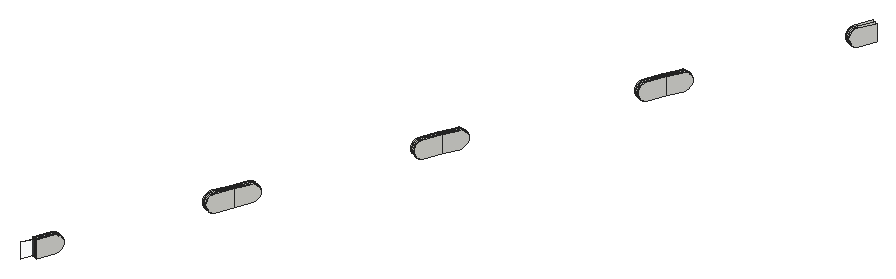
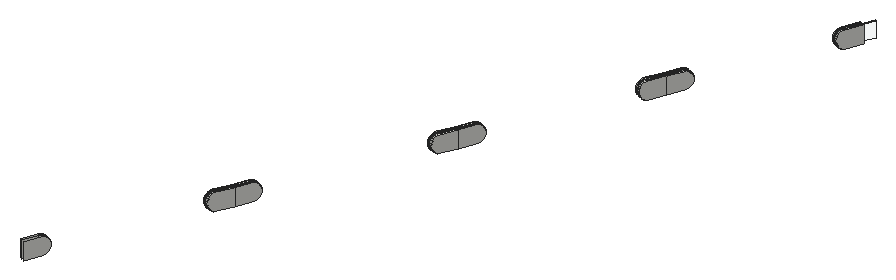
# SketchUp Ruby script. Lengths in inches.
U = 1.inch
M = Sketchup.active_model
def pt(a) = Geom::Point3d.new(a.map { |v| v * U })
def face(e, loops, mat)
  f = e.add_face(loops[0].map { |a| pt(a) })
  loops[1..].each { |l| e.add_face(l.map { |a| pt(a) }).erase! }
  f.material = f.back_material = mat if mat
  f
end
# faces: each face lists its corners as indices into pts; further lists are holes
def faces(e, pts, list, mat = nil) = list.each { |f| face(e, (f[0].is_a?(Array) ? f : [f]).map { |l| l.map { |i| pts[i] } }, mat) }
# xy, xz, yz: faces in a plane at the given z, y or x. An outline is a flat list of corners, or four numbers for a rectangle; further outlines are holes
def ring(l) = l.size == 4 ? [[l[0], l[1]], [l[2], l[1]], [l[2], l[3]], [l[0], l[3]]] : l.each_slice(2).to_a
def flat(e, list, mat, &to3) = list.each { |f| face(e, (f[0].is_a?(Array) ? f : [f]).map { |l| ring(l).map { |u, v| to3.(u, v) } }, mat) }
def xy(e, z, list, mat = nil) = flat(e, list, mat) { |x, y| [x, y, z] }
def xz(e, y, list, mat = nil) = flat(e, list, mat) { |x, z| [x, y, z] }
def yz(e, x, list, mat = nil) = flat(e, list, mat) { |y, z| [x, y, z] }
def lines(e, pts, list) = list.each { |a, b| e.add_line(pt(pts[a]), pt(pts[b])) }
# prism: a flat outline (further loops are holes) pulled along v
def prism(e, loops, v, mat = nil)
  f = face(e, loops, mat); d = Geom::Vector3d.new(v.map { |x| x * U })
  f.pushpull(f.normal.samedirection?(d) ? d.length : -d.length)
end
def box(e, o, s, mat = nil) = prism(e, [[o, [o[0] + s[0], o[1], o[2]], [o[0] + s[0], o[1] + s[1], o[2]], [o[0], o[1] + s[1], o[2]]]], [0, 0, s[2]], mat)
def at(x, y, z, deg = 0) = Geom::Transformation.translation(pt([x, y, z])) * Geom::Transformation.rotation(ORIGIN, Z_AXIS, deg.degrees)
def axes(o, x, y, z) = Geom::Transformation.new([*x, 0, *y, 0, *z, 0, *pt(o).to_a, 1])
def part(name) = M.definitions.add(name)
# library, detail: a bought-in or finely detailed component or shape, given as its bounding box
def library(name, o, s) = part(name).tap { |d| box(d.entities, o, s) }
def detail(e, o, s) = box(e.add_group.entities, o, s)
def put(e, d, t, mat = nil) = e.add_instance(d, t).tap { |i| i.material = mat if mat }
def group(e, t, mat = nil) = e.add_group.tap { |g| g.transformation = t; g.material = mat if mat }.entities
root = M.entities
M.materials.add("Glass_Safety_01").color = [204, 235, 244]
M.materials["Glass_Safety_01"].alpha = 0.1
xy(root,333,[[908.41,684.63,908.15,684.74,908.9375,686.55,909.19,686.4375],[907.97,684.82,907.72,684.93,908.51,686.74,908.76,686.625],[916.34,702.85,916.09,702.96,916.16,703.12,916.87,704.76,917.125,704.65],[915.91,703.04,915.65,703.15,916.4375,704.95,916.69,704.84,915.98,703.2],[917.125,704.65,916.87,704.76,917.66,706.57,917.91,706.46],
  [916.69,704.84,916.4375,704.95,917.23,706.76,917.48,706.65],[925.57,724.04,925.32,724.15,925.38,724.31,926.1,725.96,926.36,725.85],[925.14,724.23,924.88,724.34,925.67,726.15,925.92,726.04,925.2,724.39],[926.36,725.85,926.1,725.96,926.89,727.76,927.14,727.65],[925.92,726.04,925.67,726.15,926.46,727.95,926.71,727.84],
  [935.5,746.83,935.24,746.94,935.3,747.08,936.03,748.75,936.28,748.64],[935.0625,747.02,934.81,747.13,935.6,748.94,935.85,748.83,935.125,747.16],[936.28,748.64,936.03,748.75,936.82,750.55,937.07,750.4375],[935.85,748.83,935.6,748.94,936.39,750.74,936.64,750.63]])
xy(root,333.08,[[908.15,684.74,907.97,684.82,908.6,686.26,908.78,686.1875],[916.24,703.32,916.0625,703.4,916.69,704.84,916.87,704.76],[916.87,704.76,916.69,704.84,917.32,706.28,917.5,706.21],[925.47,724.51,925.29,724.59,925.92,726.04,926.1,725.96],[926.1,725.96,925.92,726.04,926.55,727.48,926.73,727.4],
  [935.4,747.3,935.22,747.38,935.85,748.83,935.9375,748.79,936.03,748.75],[936.03,748.75,935.9375,748.79,935.85,748.83,936.48,750.27,936.66,750.1875]],"Glass_Safety_01")
xy(root,335.05,[[907.52,683.3,908.15,684.74,907.97,684.82,907.34,683.375],[908.15,684.74,908.78,686.1875,908.6,686.26,907.97,684.82],[916.24,703.32,916.87,704.76,916.69,704.84,916.0625,703.4],[916.87,704.76,917.5,706.21,917.32,706.28,916.69,704.84],[925.47,724.51,926.1,725.96,925.92,726.04,925.29,724.59],
  [926.1,725.96,926.73,727.4,926.55,727.48,925.92,726.04],[935.4,747.3,936.03,748.75,935.9375,748.79,935.85,748.83,935.22,747.38],[936.03,748.75,936.66,750.1875,936.48,750.27,935.85,748.83,935.9375,748.79]],"Glass_Safety_01")
xy(root,335.125,[[908.41,684.63,909.19,686.4375,908.9375,686.55,908.15,684.74],[907.97,684.82,908.76,686.625,908.51,686.74,907.72,684.93],[916.34,702.85,917.125,704.65,916.87,704.76,916.16,703.12,916.09,702.96],[915.91,703.04,915.98,703.2,916.69,704.84,916.4375,704.95,915.65,703.15],[917.125,704.65,917.91,706.46,917.66,706.57,916.87,704.76],
  [916.69,704.84,917.48,706.65,917.23,706.76,916.4375,704.95],[925.57,724.04,926.36,725.85,926.1,725.96,925.38,724.31,925.32,724.15],[925.14,724.23,925.2,724.39,925.92,726.04,925.67,726.15,924.88,724.34],[926.36,725.85,927.14,727.65,926.89,727.76,926.1,725.96],[925.92,726.04,926.71,727.84,926.46,727.95,925.67,726.15],
  [935.5,746.83,936.28,748.64,936.03,748.75,935.3,747.08,935.24,746.94],[935.0625,747.02,935.125,747.16,935.85,748.83,935.6,748.94,934.81,747.13],[936.28,748.64,937.07,750.4375,936.82,750.55,936.03,748.75],[935.85,748.83,936.64,750.63,936.39,750.74,935.6,748.94]])
p = [[908.15,684.74,333],[908.15,684.74,333.08],[908.15,684.74,335.05],[908.15,684.74,335.125],[908.41,684.63,335.125],[908.41,684.63,333],
  [909.19,686.4375,335.125],[909.19,686.4375,333],[909.3,686.6875,333.04],[909.4,686.92,333.14],[909.49,687.125,333.3125],[909.56,687.28,333.53],
  [909.6,687.38,333.79],[909.62,687.41,334.0625],[909.6,687.38,334.34],[909.56,687.28,334.59],[909.49,687.125,334.8125],[909.4,686.92,334.98],
  [909.3,686.6875,335.09],[908.9375,686.55,335.125],[908.9375,686.55,333],[908.78,686.1875,333.08],[908.78,686.1875,335.05],[907.97,684.82,333.08],
  [907.97,684.82,333],[907.72,684.93,333],[907.72,684.93,335.125],[907.97,684.82,335.125],[907.97,684.82,335.05],[908.76,686.625,333],
  [908.76,686.625,335.125],[908.6,686.26,335.05],[908.6,686.26,333.08],[908.51,686.74,335.125],[908.62,686.99,335.09],[908.72,687.22,334.98],
  [908.81,687.42,334.8125],[908.875,687.58,334.59],[908.92,687.68,334.34],[908.93,687.71,334.0625],[908.92,687.68,333.79],[908.875,687.58,333.53],
  [908.81,687.42,333.3125],[908.72,687.22,333.14],[908.62,686.99,333.04],[908.51,686.74,333],[909.05,686.8,333.04],[909.15,687.03,333.14],
  [909.24,687.24,333.3125],[909.31,687.39,333.53],[909.35,687.49,333.79],[909.36,687.52,334.0625],[909.35,687.49,334.34],[909.31,687.39,334.59],
  [909.24,687.24,334.8125],[909.15,687.03,334.98],[909.05,686.8,335.09],[908.87,686.88,333.04],[908.87,686.88,335.09],[908.97,687.11,334.98],
  [909.06,687.3125,334.8125],[909.125,687.47,334.59],[909.17,687.57,334.34],[909.18,687.6,334.0625],[909.17,687.57,333.79],[909.125,687.47,333.53],
  [909.06,687.3125,333.3125],[908.97,687.11,333.14],[917.125,704.65,335.125],[916.34,702.85,335.125],[916.23,702.6,335.09],[916.125,702.36,334.98],
  [916.04,702.16,334.8125],[915.97,702,334.59],[915.93,701.91,334.34],[915.91,701.875,334.0625],[915.93,701.91,333.79],[915.97,702,333.53],
  [916.04,702.16,333.3125],[916.125,702.36,333.14],[916.23,702.6,333.04],[916.34,702.85,333],[917.125,704.65,333],[916.09,702.96,335.125],
  [916.16,703.12,335.125],[916.16,703.12,333],[916.09,702.96,333],[915.98,702.71,333.04],[915.875,702.47,333.14],[915.79,702.27,333.3125],
  [915.72,702.11,333.53],[915.68,702.02,333.79],[915.66,701.98,334.0625],[915.68,702.02,334.34],[915.72,702.11,334.59],[915.79,702.27,334.8125],
  [915.875,702.47,334.98],[915.98,702.71,335.09],[915.91,703.04,333],[915.98,703.2,333],[915.98,703.2,335.125],[915.91,703.04,335.125],
  [915.8,702.78,335.09],[915.69,702.55,334.98],[915.61,702.35,334.8125],[915.54,702.19,334.59],[915.5,702.1,334.34],[915.48,702.0625,334.0625],
  [915.5,702.1,333.79],[915.54,702.19,333.53],[915.61,702.35,333.3125],[915.69,702.55,333.14],[915.8,702.78,333.04],[915.65,703.15,335.125],
  [916.4375,704.95,335.125],[916.4375,704.95,333],[915.65,703.15,333],[915.54,702.89,333.04],[915.44,702.66,333.14],[915.35,702.46,333.3125],
  [915.29,702.3,333.53],[915.24,702.21,333.79],[915.23,702.17,334.0625],[915.24,702.21,334.34],[915.29,702.3,334.59],[915.35,702.46,334.8125],
  [915.44,702.66,334.98],[915.54,702.89,335.09],[916.87,704.76,333],[916.87,704.76,335.125],[916.87,704.76,335.05],[916.24,703.32,335.05],
  [916.24,703.32,333.08],[916.87,704.76,333.08],[916.69,704.84,335.125],[916.69,704.84,333],[916.69,704.84,333.08],[916.0625,703.4,333.08],
  [916.0625,703.4,335.05],[916.69,704.84,335.05],[917.91,706.46,335.125],[917.91,706.46,333],[918.02,706.71,333.04],[918.125,706.94,333.14],
  [918.21,707.15,333.3125],[918.28,707.3,333.53],[918.32,707.4,333.79],[918.34,707.43,334.0625],[918.32,707.4,334.34],[918.28,707.3,334.59],
  [918.21,707.15,334.8125],[918.125,706.94,334.98],[918.02,706.71,335.09],[917.48,706.65,333],[917.48,706.65,335.125],[917.32,706.28,335.05],
  [917.32,706.28,333.08],[917.66,706.57,335.125],[917.66,706.57,333],[917.5,706.21,333.08],[917.5,706.21,335.05],[917.23,706.76,335.125],
  [917.33,707.01,335.09],[917.4375,707.24,334.98],[917.53,707.45,334.8125],[917.59,707.6,334.59],[917.64,707.7,334.34],[917.65,707.73,334.0625],
  [917.64,707.7,333.79],[917.59,707.6,333.53],[917.53,707.45,333.3125],[917.4375,707.24,333.14],[917.33,707.01,333.04],[917.23,706.76,333],
  [917.77,706.82,333.04],[917.59,706.9,333.04],[917.59,706.9,335.09],[917.69,707.13,334.98],[917.78,707.34,334.8125],[917.85,707.49,334.59],
  [917.89,707.59,334.34],[917.9,707.62,334.0625],[917.89,707.59,333.79],[917.85,707.49,333.53],[917.78,707.34,333.3125],[917.69,707.13,333.14],
  [917.87,707.05,333.14],[917.96,707.26,333.3125],[918.03,707.41,333.53],[918.07,707.51,333.79],[918.08,707.54,334.0625],[918.07,707.51,334.34],
  [918.03,707.41,334.59],[917.96,707.26,334.8125],[917.87,707.05,334.98],[917.77,706.82,335.09],[926.36,725.85,335.125],[925.57,724.04,335.125],
  [925.46,723.79,335.09],[925.36,723.56,334.98],[925.27,723.35,334.8125],[925.2,723.2,334.59],[925.16,723.1,334.34],[925.15,723.07,334.0625],
  [925.16,723.1,333.79],[925.2,723.2,333.53],[925.27,723.35,333.3125],[925.36,723.56,333.14],[925.46,723.79,333.04],[925.57,724.04,333],
  [926.36,725.85,333],[925.32,724.15,335.125],[925.38,724.31,335.125],[925.38,724.31,333],[925.32,724.15,333],[925.21,723.9,333.04],
  [925.11,723.67,333.14],[925.02,723.46,333.3125],[924.95,723.31,333.53],[924.91,723.21,333.79],[924.89,723.18,334.0625],[924.91,723.21,334.34],
  [924.95,723.31,334.59],[925.02,723.46,334.8125],[925.11,723.67,334.98],[925.21,723.9,335.09],[925.14,724.23,333],[925.2,724.39,333],
  [925.2,724.39,335.125],[925.14,724.23,335.125],[925.03,723.98,335.09],[924.92,723.74,334.98],[924.84,723.54,334.8125],[924.77,723.39,334.59],
  [924.73,723.29,334.34],[924.71,723.26,334.0625],[924.73,723.29,333.79],[924.77,723.39,333.53],[924.84,723.54,333.3125],[924.92,723.74,333.14],
  [925.03,723.98,333.04],[924.88,724.34,335.125],[925.67,726.15,335.125],[925.67,726.15,333],[924.88,724.34,333],[924.77,724.09,333.04],
  [924.67,723.85,333.14],[924.58,723.65,333.3125],[924.52,723.5,333.53],[924.47,723.4,333.79],[924.46,723.37,334.0625],[924.47,723.4,334.34],
  [924.52,723.5,334.59],[924.58,723.65,334.8125],[924.67,723.85,334.98],[924.77,724.09,335.09],[926.1,725.96,333],[926.1,725.96,335.125],
  [926.1,725.96,335.05],[925.47,724.51,335.05],[925.47,724.51,333.08],[926.1,725.96,333.08],[925.92,726.04,335.125],[925.92,726.04,333],
  [925.92,726.04,333.08],[925.29,724.59,333.08],[925.29,724.59,335.05],[925.92,726.04,335.05],[927.14,727.65,335.125],[927.14,727.65,333],
  [927.25,727.91,333.04],[927.35,728.14,333.14],[927.44,728.34,333.3125],[927.51,728.5,333.53],[927.55,728.59,333.79],[927.57,728.63,334.0625],
  [927.55,728.59,334.34],[927.51,728.5,334.59],[927.44,728.34,334.8125],[927.35,728.14,334.98],[927.25,727.91,335.09],[926.71,727.84,333],
  [926.71,727.84,335.125],[926.55,727.48,335.05],[926.55,727.48,333.08],[926.89,727.76,335.125],[926.89,727.76,333],[926.73,727.4,333.08],
  [926.73,727.4,335.05],[926.46,727.95,335.125],[926.57,728.2,335.09],[926.67,728.4375,334.98],[926.76,728.64,334.8125],[926.82,728.8,334.59],
  [926.87,728.89,334.34],[926.88,728.93,334.0625],[926.87,728.89,333.79],[926.82,728.8,333.53],[926.76,728.64,333.3125],[926.67,728.4375,333.14],
  [926.57,728.2,333.04],[926.46,727.95,333],[927,728.02,333.04],[926.82,728.09,333.04],[926.82,728.09,335.09],[926.92,728.33,334.98],
  [927.01,728.53,334.8125],[927.08,728.6875,334.59],[927.12,728.78,334.34],[927.13,728.82,334.0625],[927.12,728.78,333.79],[927.08,728.6875,333.53],
  [927.01,728.53,333.3125],[926.92,728.33,333.14],[927.1,728.25,333.14],[927.19,728.45,333.3125],[927.26,728.61,333.53],[927.3,728.7,333.79],
  [927.3125,728.74,334.0625],[927.3,728.7,334.34],[927.26,728.61,334.59],[927.19,728.45,334.8125],[927.1,728.25,334.98],[927,728.02,335.09],
  [936.28,748.64,335.125],[935.5,746.83,335.125],[935.39,746.58,335.09],[935.28,746.34,334.98],[935.2,746.14,334.8125],[935.13,745.99,334.59],
  [935.09,745.89,334.34],[935.07,745.86,334.0625],[935.09,745.89,333.79],[935.13,745.99,333.53],[935.2,746.14,333.3125],[935.28,746.34,333.14],
  [935.39,746.58,333.04],[935.5,746.83,333],[936.28,748.64,333],[935.0625,747.02,333],[935.125,747.16,333],[935.125,747.16,335.125],
  [935.0625,747.02,335.125],[934.95,746.77,335.09],[934.85,746.53,334.98],[934.76,746.33,334.8125],[934.69,746.18,334.59],[934.65,746.08,334.34],
  [934.64,746.05,334.0625],[934.65,746.08,333.79],[934.69,746.18,333.53],[934.76,746.33,333.3125],[934.85,746.53,333.14],[934.95,746.77,333.04],
  [935.24,746.94,335.125],[935.3,747.08,335.125],[935.3,747.08,333],[935.24,746.94,333],[935.13,746.69,333.04],[935.03,746.45,333.14],
  [934.94,746.25,333.3125],[934.875,746.1,333.53],[934.83,746,333.79],[934.82,745.97,334.0625],[934.83,746,334.34],[934.875,746.1,334.59],
  [934.94,746.25,334.8125],[935.03,746.45,334.98],[935.13,746.69,335.09],[934.81,747.13,335.125],[935.6,748.94,335.125],[935.6,748.94,333],
  [934.81,747.13,333],[934.7,746.88,333.04],[934.6,746.64,333.14],[934.51,746.44,333.3125],[934.44,746.29,333.53],[934.4,746.1875,333.79],
  [934.38,746.16,334.0625],[934.4,746.1875,334.34],[934.44,746.29,334.59],[934.51,746.44,334.8125],[934.6,746.64,334.98],[934.7,746.88,335.09],
  [936.03,748.75,333],[936.03,748.75,335.125],[936.03,748.75,335.05],[935.4,747.3,335.05],[935.4,747.3,333.08],[936.03,748.75,333.08],
  [935.85,748.83,335.125],[935.85,748.83,333],[935.85,748.83,333.08],[935.22,747.38,333.08],[935.22,747.38,335.05],[935.85,748.83,335.05],
  [937.07,750.4375,335.125],[937.07,750.4375,333],[937.18,750.6875,333.04],[937.29,750.92,333.14],[937.375,751.125,333.3125],[937.44,751.28,333.53],
  [937.49,751.38,333.79],[937.5,751.41,334.0625],[937.49,751.38,334.34],[937.44,751.28,334.59],[937.375,751.125,334.8125],[937.29,750.92,334.98],
  [937.18,750.6875,335.09],[936.82,750.55,335.125],[936.82,750.55,333],[936.66,750.1875,333.08],[936.66,750.1875,335.05],[936.64,750.63,333],
  [936.64,750.63,335.125],[936.48,750.27,335.05],[936.48,750.27,333.08],[936.39,750.74,335.125],[936.5,750.99,335.09],[936.6,751.23,334.98],
  [936.69,751.43,334.8125],[936.76,751.58,334.59],[936.8,751.68,334.34],[936.82,751.71,334.0625],[936.8,751.68,333.79],[936.76,751.58,333.53],
  [936.69,751.43,333.3125],[936.6,751.23,333.14],[936.5,750.99,333.04],[936.39,750.74,333],[936.93,750.8,333.04],[937.03,751.03,333.14],
  [937.125,751.24,333.3125],[937.19,751.39,333.53],[937.23,751.49,333.79],[937.25,751.52,334.0625],[937.23,751.49,334.34],[937.19,751.39,334.59],
  [937.125,751.24,334.8125],[937.03,751.03,334.98],[936.93,750.8,335.09],[936.75,750.88,333.04],[936.75,750.88,335.09],[936.85,751.11,334.98],
  [936.94,751.32,334.8125],[937.01,751.47,334.59],[937.05,751.57,334.34],[937.07,751.6,334.0625],[937.05,751.57,333.79],[937.01,751.47,333.53],
  [936.94,751.32,333.3125],[936.85,751.11,333.14],[944.88,768.2,333],[945.67,769.99,333],[945.67,769.99,335.125],[944.88,768.2,335.125],
  [944.77,767.95,335.09],[944.67,767.72,334.98],[944.58,767.51,334.8125],[944.51,767.36,334.59],[944.47,767.26,334.34],[944.46,767.23,334.0625],
  [944.47,767.26,333.79],[944.51,767.36,333.53],[944.58,767.51,333.3125],[944.67,767.72,333.14],[944.77,767.95,333.04],[944.7,768.46,335.125],
  [945.42,770.11,335.125],[945.42,770.11,335.05],[945.42,770.11,333.08],[945.42,770.11,333],[944.7,768.46,333],[944.63,768.3125,333],
  [944.52,768.0625,333.04],[944.42,767.83,333.14],[944.33,767.625,333.3125],[944.26,767.47,333.53],[944.22,767.37,333.79],[944.2,767.34,334.0625],
  [944.22,767.37,334.34],[944.26,767.47,334.59],[944.33,767.625,334.8125],[944.42,767.83,334.98],[944.52,768.0625,335.09],[944.63,768.3125,335.125],
  [944.45,768.39,333],[944.52,768.54,333],[944.52,768.54,335.125],[944.45,768.39,335.125],[944.34,768.14,335.09],[944.24,767.91,334.98],
  [944.15,767.7,334.8125],[944.08,767.55,334.59],[944.04,767.45,334.34],[944.02,767.42,334.0625],[944.04,767.45,333.79],[944.08,767.55,333.53],
  [944.15,767.7,333.3125],[944.24,767.91,333.14],[944.34,768.14,333.04],[944.2,768.5,335.125],[944.99,770.3,335.125],[944.99,770.3,333],
  [944.2,768.5,333],[944.09,768.25,333.04],[943.99,768.02,333.14],[943.9,767.81,333.3125],[943.83,767.66,333.53],[943.79,767.5625,333.79],
  [943.77,767.53,334.0625],[943.79,767.5625,334.34],[943.83,767.66,334.59],[943.9,767.81,334.8125],[943.99,768.02,334.98],[944.09,768.25,335.09],
  [907.34,683.375,333.08],[907.34,683.375,335.05],[935.9375,748.79,333.08],[935.9375,748.79,335.05]]
faces(root,p,[[0,1,2,3,4,5],[6,4,5,7,8,9,10,11,12,13,14,15,16,17,18],[3,19,20,0,1,21,22,2],[23,24,25,26,27,28],[24,29,30,27,28,31,32,23],[26,33,34,35,36,37,38,39,40,41,42,43,44,45,25],[20,46,8,7],[57,29,45,44],
  [46,47,9,8],[67,57,44,43],[68,69,70,71,72,73,74,75,76,77,78,79,80,81,82],[83,84,85,86,87,88,89,90,91,92,93,94,95,96,97],[98,99,100,101,102,103,104,105,106,107,108,109,110,111,112],[113,114,115,116,117,118,119,120,121,122,123,124,125,126,127],[88,87,80,79],[112,111,118,117],
  [87,86,81,80],[98,112,117,116],[128,85,84,129,130,131,132,133],[134,100,99,135,136,137,138,139],[128,133,130,129,68,82],[140,68,82,141,142,143,144,145,146,147,148,149,150,151,152],[136,135,115,114,134,139],[135,153,154,134,139,155,156,136],
  [129,157,158,128,133,159,160,130],[114,161,162,163,164,165,166,167,168,169,170,171,172,173,115],[158,174,142,141],[175,153,173,172],[174,186,143,142],[185,175,172,171],[196,197,198,199,200,201,202,203,204,205,206,207,208,209,210],[211,212,213,214,215,216,217,218,219,220,221,222,223,224,225],
  [226,227,228,229,230,231,232,233,234,235,236,237,238,239,240],[241,242,243,244,245,246,247,248,249,250,251,252,253,254,255],[216,215,208,207],[240,239,246,245],[215,214,209,208],[226,240,245,244],[256,213,212,257,258,259,260,261],[262,228,227,263,264,265,266,267],
  [256,261,258,257,196,210],[268,196,210,269,270,271,272,273,274,275,276,277,278,279,280],[264,263,243,242,262,267],[263,281,282,262,267,283,284,264],[257,285,286,256,261,287,288,258],[242,289,290,291,292,293,294,295,296,297,298,299,300,301,243],[286,302,270,269],[303,281,301,300],
  [302,314,271,270],[313,303,300,299],[324,325,326,327,328,329,330,331,332,333,334,335,336,337,338],[339,340,341,342,343,344,345,346,347,348,349,350,351,352,353],[354,355,356,357,358,359,360,361,362,363,364,365,366,367,368],[369,370,371,372,373,374,375,376,377,378,379,380,381,382,383],[359,358,336,335],[353,352,374,373],
  [358,357,337,336],[339,353,373,372],[384,356,355,385,386,387,388,389],[390,341,340,391,392,393,394,395],[384,389,386,385,324,338],[396,324,338,397,398,399,400,401,402,403,404,405,406,407,408],[385,409,410,384,389,411,412,386],[392,391,371,370,390,395],
  [391,413,414,390,395,415,416,392],[370,417,418,419,420,421,422,423,424,425,426,427,428,429,371],[410,430,398,397],[441,413,429,428],[430,431,399,398],[451,441,428,427],[452,453,454,455,456,457,458,459,460,461,462,463,464,465,466],[467,468,469,470,471,472,473,474,475,476,477,478,479,480,481,482,483,484,485],
  [486,487,488,489,490,491,492,493,494,495,496,497,498,499,500],[501,502,503,504,505,506,507,508,509,510,511,512,513,514,515],[475,474,466,465],[500,499,506,505],[474,473,452,466],[47,48,10,9],[66,67,43,42],[89,88,79,78],
  [111,110,119,118],[186,187,144,143],[184,185,171,170],[217,216,207,206],[239,238,247,246],[314,315,272,271],[312,313,299,298],[360,359,335,334],
  [352,351,375,374],[431,432,400,399],[450,451,427,426],[476,475,465,464],[499,498,507,506],[48,49,11,10],[65,66,42,41],[90,89,78,77],
  [110,109,120,119],[187,188,145,144],[183,184,170,169],[218,217,206,205],[238,237,248,247],[315,316,273,272],[311,312,298,297],[361,360,334,333],
  [351,350,376,375],[432,433,401,400],[449,450,426,425],[477,476,464,463],[498,497,508,507],[49,50,12,11],[64,65,41,40],[91,90,77,76],
  [109,108,121,120],[188,189,146,145],[182,183,169,168],[219,218,205,204],[237,236,249,248],[316,317,274,273],[310,311,297,296],[362,361,333,332],
  [350,349,377,376],[433,434,402,401],[448,449,425,424],[478,477,463,462],[497,496,509,508],[50,51,13,12],[63,64,40,39],[92,91,76,75],
  [108,107,122,121],[189,190,147,146],[181,182,168,167],[220,219,204,203],[236,235,250,249],[317,318,275,274],[309,310,296,295],[363,362,332,331],
  [349,348,378,377],[434,435,403,402],[447,448,424,423],[479,478,462,461],[496,495,510,509],[51,52,14,13],[62,63,39,38],[93,92,75,74],
  [107,106,123,122],[190,191,148,147],[180,181,167,166],[221,220,203,202],[235,234,251,250],[318,319,276,275],[308,309,295,294],[364,363,331,330],
  [348,347,379,378],[435,436,404,403],[446,447,423,422],[480,479,461,460],[495,494,511,510],[52,53,15,14],[61,62,38,37],[94,93,74,73],
  [106,105,124,123],[191,192,149,148],[179,180,166,165],[222,221,202,201],[234,233,252,251],[319,320,277,276],[307,308,294,293],[365,364,330,329],
  [347,346,380,379],[436,437,405,404],[445,446,422,421],[481,480,460,459],[494,493,512,511],[53,54,16,15],[60,61,37,36],[95,94,73,72],
  [105,104,125,124],[192,193,150,149],[178,179,165,164],[223,222,201,200],[233,232,253,252],[320,321,278,277],[306,307,293,292],[366,365,329,328],
  [346,345,381,380],[437,438,406,405],[444,445,421,420],[482,481,459,458],[493,492,513,512],[54,55,17,16],[59,60,36,35],[96,95,72,71],
  [104,103,126,125],[193,194,151,150],[177,178,164,163],[224,223,200,199],[232,231,254,253],[321,322,279,278],[305,306,292,291],[367,366,328,327],
  [345,344,382,381],[438,439,407,406],[443,444,420,419],[483,482,458,457],[492,491,514,513],[55,56,18,17],[58,59,35,34],[97,96,71,70],
  [103,102,127,126],[194,195,152,151],[176,177,163,162],[225,224,199,198],[231,230,255,254],[322,323,280,279],[304,305,291,290],[368,367,327,326],
  [344,343,383,382],[439,440,408,407],[442,443,419,418],[484,483,457,456],[491,490,515,514],[56,19,6,18],[30,58,34,33],[83,97,70,69],
  [102,101,113,127],[195,157,140,152],[154,176,162,161],[211,225,198,197],[230,229,241,255],[323,285,268,280],[282,304,290,289],[354,368,326,325],
  [343,342,369,383],[440,409,396,408],[414,442,418,417],[485,484,456,455]])
faces(root,p,[[19,20,46,47,48,49,50,51,52,53,54,55,56],[29,30,58,59,60,61,62,63,64,65,66,67,57],[153,154,176,177,178,179,180,181,182,183,184,185,175],[157,158,174,186,187,188,189,190,191,192,193,194,195],[281,282,304,305,306,307,308,309,310,311,312,313,303],[285,286,302,314,315,316,317,318,319,320,321,322,323],[409,410,430,431,432,433,434,435,436,437,438,439,440],[413,414,442,443,444,445,446,447,448,449,450,451,441],
  [516,23,28,517],[28,2,1,23],[21,1,2,22],[23,32,31,28],[22,21,32,31],[132,131,138,137],[133,132,131,130],[137,136,139,138],
  [139,130,133,136],[136,156,155,139],[159,133,130,160],[160,159,156,155],[260,259,266,265],[261,260,259,258],[265,264,267,266],[267,258,261,264],
  [264,284,283,267],[287,261,258,288],[288,287,284,283],[388,387,394,393],[389,388,387,386],[393,392,395,394],[389,518,519,386],[411,389,386,412],
  [395,519,518,392],[392,416,415,395],[415,412,411,416]],"Glass_Safety_01")
